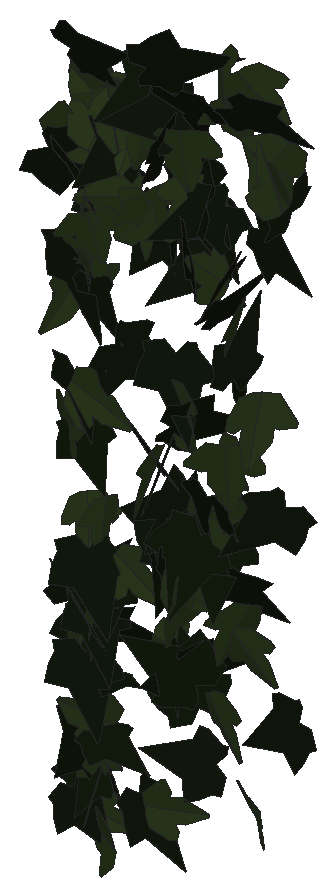
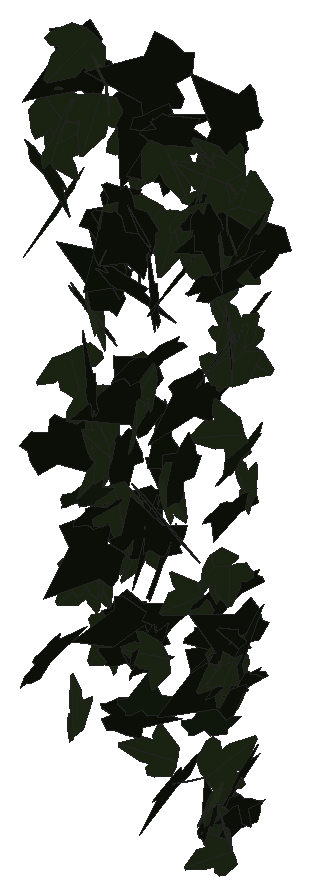
# SketchUp Ruby script. Lengths in inches.
U = 1.inch
M = Sketchup.active_model
def pt(a) = Geom::Point3d.new(a.map { |v| v * U })
def face(e, loops, mat)
  f = e.add_face(loops[0].map { |a| pt(a) })
  loops[1..].each { |l| e.add_face(l.map { |a| pt(a) }).erase! }
  f.material = f.back_material = mat if mat
  f
end
# faces: each face lists its corners as indices into pts; further lists are holes
def faces(e, pts, list, mat = nil) = list.each { |f| face(e, (f[0].is_a?(Array) ? f : [f]).map { |l| l.map { |i| pts[i] } }, mat) }
# xy, xz, yz: faces in a plane at the given z, y or x. An outline is a flat list of corners, or four numbers for a rectangle; further outlines are holes
def ring(l) = l.size == 4 ? [[l[0], l[1]], [l[2], l[1]], [l[2], l[3]], [l[0], l[3]]] : l.each_slice(2).to_a
def flat(e, list, mat, &to3) = list.each { |f| face(e, (f[0].is_a?(Array) ? f : [f]).map { |l| ring(l).map { |u, v| to3.(u, v) } }, mat) }
def xy(e, z, list, mat = nil) = flat(e, list, mat) { |x, y| [x, y, z] }
def xz(e, y, list, mat = nil) = flat(e, list, mat) { |x, z| [x, y, z] }
def yz(e, x, list, mat = nil) = flat(e, list, mat) { |y, z| [x, y, z] }
def lines(e, pts, list) = list.each { |a, b| e.add_line(pt(pts[a]), pt(pts[b])) }
# prism: a flat outline (further loops are holes) pulled along v
def prism(e, loops, v, mat = nil)
  f = face(e, loops, mat); d = Geom::Vector3d.new(v.map { |x| x * U })
  f.pushpull(f.normal.samedirection?(d) ? d.length : -d.length)
end
def box(e, o, s, mat = nil) = prism(e, [[o, [o[0] + s[0], o[1], o[2]], [o[0] + s[0], o[1] + s[1], o[2]], [o[0], o[1] + s[1], o[2]]]], [0, 0, s[2]], mat)
def at(x, y, z, deg = 0) = Geom::Transformation.translation(pt([x, y, z])) * Geom::Transformation.rotation(ORIGIN, Z_AXIS, deg.degrees)
def axes(o, x, y, z) = Geom::Transformation.new([*x, 0, *y, 0, *z, 0, *pt(o).to_a, 1])
def part(name) = M.definitions.add(name)
# library, detail: a bought-in or finely detailed component or shape, given as its bounding box
def library(name, o, s) = part(name).tap { |d| box(d.entities, o, s) }
def detail(e, o, s) = box(e.add_group.entities, o, s)
def put(e, d, t, mat = nil) = e.add_instance(d, t).tap { |i| i.material = mat if mat }
def group(e, t, mat = nil) = e.add_group.tap { |g| g.transformation = t; g.material = mat if mat }.entities
root = M.entities
M.materials.add("efeu1").color = [18, 25, 13]
M.materials.add("efeu2").color = [43, 57, 29]
c1 = part("ivyleaf_10")
p = [[0,0.5,-0.03],[-0.0625,2.02,-0.43],[-0.19,2.01,-0.46],[-0.54,1.05,-0.29],[-0.52,0.625,-0.18],[-0.83,0.76,-0.28],
  [-1.16,0.64,-0.33],[-1.15,0.33,-0.24],[-0.77,-0.39,0.02],[-0.3,-0.51,0.16],[0.04,-0.48,0.23],[-0.02,2.01,-0.4375],
  [-0.06,2.01,-0.43],[0.04,-0.49,0.23],[0.67,-0.49,0.14],[1.38,0.36,-0.2],[1.375,0.51,-0.24],[0.81,0.65,-0.19],
  [0.62,0.59,-0.15],[0.6,1.09,-0.28],[0.5,1.23,-0.31]]
faces(c1.entities,p,[[0,1,2,3,4,5,6,7,8,9,10],[11,12,0,13,14,15,16,17,18,19,20]],"efeu2")
c2 = part("ivyleaf_9")
p = [[1.54,2.16,1.25],[1.36,2.04,1.19],[-0.21,0.99,0.68],[-0.71,1.11,0.82],[-0.85,0.86,0.67],[-0.8,0.17,0.21],
  [-0.9,-0.01,0.1],[-0.67,-0.16,-0.02],[-0.08,-0.08,-0.05],[-0.03,-0.6,-0.4],[0.65,-0.88,-0.66],[0.83,-0.6,-0.49],
  [1.29,-0.42,-0.43],[1.8125,-0.07,-0.26],[1.21,0.44,0.15]]
faces(c2.entities,p,[[0,1,2,3,4,5,6,7,8,9,10,11,12,13,14]],"efeu1")
put(root,c1,axes([585.43,126.89,216.26],[0.20905,0.88225,-0.1568],[-0.02786,-0.15453,-0.90664],[-0.89564,0.21074,-0.00839]))
put(root,c1,axes([585.7,127.05,216.36],[-0.86933,0.26454,0.1104],[-0.10638,0.02961,-0.90868],[-0.26618,-0.87581,0.00262]))
put(root,c2,axes([586.2,127.75,234.65],[-0.4505,-1.00807,-0.18395],[-0.0756,-0.1677,1.10415],[-1.02192,0.4568,-0.00059]))
put(root,c1,axes([585.82,126.15,231.04],[0.26542,0.80579,-0.93729],[-0.44182,-0.83347,-0.84165],[-1.15439,0.50427,0.10662]))
put(root,c1,axes([586.16,127.11,211.16],[-0.42988,-0.39281,-0.89243],[-0.69049,-0.56599,0.58173],[-0.68844,0.81295,-0.02621]))
put(root,c2,axes([585.43,126.77,210.41],[-0.05024,-0.67641,0.89624],[-0.10277,-0.89061,-0.67792],[1.11814,-0.11225,-0.02203]))
put(root,c2,axes([585.53,126.99,215.375],[-0.24572,-0.87489,-0.04621],[0.01577,0.04356,-0.90873],[0.87597,-0.2462,0.0034]))
put(root,c2,axes([585.18,126.625,226.41],[0.33854,-0.96981,0.40729],[0.20018,-0.36064,-1.02513],[1.03264,0.38786,0.0652]))
put(root,c1,axes([585.7,126.66,230.41],[-0.41477,-1.0757,-0.15207],[-0.02291,-0.15408,1.1524],[-1.08615,0.41403,0.03377]))
put(root,c1,axes([585.64,126.8125,220.75],[0.5479,0.75565,-0.02304],[-0.01674,-0.01633,-0.93337],[-0.75581,0.54814,0.00396]))
put(root,c1,axes([585.18,126.07,224.39],[-0.45576,0.14929,0.94388],[0.90384,-0.27221,0.47948],[0.31029,1.01219,-0.01027]))
put(root,c2,axes([586.03,126.6875,215.52],[0.58846,-0.99171,0.4904],[-0.25923,0.41639,1.15312],[-1.07554,-0.64296,-0.00962]))
put(root,c2,axes([585.51,126.76,224.1],[0.1079,-0.87299,-0.38514],[-0.01408,0.3861,-0.8791],[0.95407,0.10443,0.03058]))
put(root,c2,axes([585.39,127.19,232.5],[-0.23152,-0.02001,-1.13527],[1.10371,-0.27602,-0.22022],[-0.2666,-1.12528,0.07421]))
put(root,c2,axes([585.27,125.92,236.77],[0.54697,-0.82406,0.44768],[0.24394,-0.3754,-0.98906],[0.90553,0.59889,-0.00397]))
put(root,c2,axes([585.26,125.15,237.09],[0.09927,0.31832,-1.30453],[0.49473,1.20741,0.33226],[1.24835,-0.50381,-0.02794]))
put(root,c2,axes([585.64,125.9,217.02],[-0.10869,-0.07593,1.08353],[0.91589,0.57898,0.13245],[-0.5839,0.92229,0.00606]))
put(root,c2,axes([586.07,126.57,209.21],[-0.52865,-0.66925,0.02633],[-0.01514,-0.02159,-0.85285],[0.6696,-0.52886,0.0015]))
put(root,c1,axes([585.75,126.25,231.91],[-0.81,-0.25854,0.56525],[0.53534,0.18165,0.85022],[-0.31586,0.97088,-0.00855]))
put(root,c1,axes([585.71,126.32,231.35],[-0.61315,0.22458,0.77909],[0.70857,-0.32642,0.65173],[0.39416,0.93615,0.04035]))
put(root,c1,axes([586.16,126.68,208.8],[0.65539,-0.82227,0.0305],[0.01965,-0.02334,-1.05151],[0.8226,0.65568,0.00082]))
put(root,c1,axes([585.98,126.27,216.35],[-0.35302,-0.53148,-0.79615],[0.41333,0.68076,-0.63772],[0.86342,-0.54319,-0.02023]))
put(root,c2,axes([585.52,125.85,232.41],[0.61194,-1.20843,0.05809],[0.0345,-0.04764,-1.35451],[1.20934,0.61284,0.00924]))
put(root,c1,axes([585.47,125.34,237.7],[-0.1941,-0.30638,1.14812],[0.86858,0.75731,0.34894],[-0.81093,0.88449,0.09894]))
put(root,c2,axes([586.75,127.12,237.64],[0.37189,0.07914,-1.04316],[-1.03126,-0.15844,-0.37967],[-0.17592,1.09607,0.02043]))
put(root,c2,axes([585.9,125.73,208.58],[0.27516,-0.71599,-0.67061],[-0.14859,0.65804,-0.76353],[0.96968,0.304,0.0733]))
put(root,c1,axes([586.15,127.01,209.59],[-0.04471,-0.90231,0.11582],[0.22003,-0.12324,-0.8752],[0.8827,-0.01499,0.22403]))
put(root,c1,axes([586.45,126.43,236.62],[0.21412,-1.02771,-0.08026],[-0.01363,0.07915,-1.04978],[1.03075,0.21454,0.00279]))
put(root,c1,axes([586.16,126.98,210.19],[0.54963,-0.61414,-0.27508],[0.28349,0.53344,-0.6245],[0.6103,0.3053,0.53783]))
put(root,c1,axes([585.85,126.98,207.12],[0.31525,0.16728,0.79766],[0.58161,0.55295,-0.34583],[-0.57093,0.65566,0.08814]))
put(root,c2,axes([585.91,126.64,215.5],[0.83714,0.54152,0.56986],[0.47909,0.30855,-0.99702],[-0.62325,0.96454,-0.00099]))
put(root,c1,axes([586.46,126.82,220.84],[-0.04804,-0.94628,0.20964],[0.23662,-0.215,-0.91624],[0.9399,0.00576,0.24138]))
put(root,c2,axes([586.42,126.95,217.52],[-0.52671,-0.6679,-0.42065],[0.24692,0.3409,-0.85045],[0.74971,-0.58151,-0.01542]))
put(root,c1,axes([586.29,126.48,216.25],[0.25401,-0.57922,0.64008],[0.49141,-0.45154,-0.60362],[0.70973,0.51994,0.18885]))
put(root,c2,axes([586.17,127.56,208.73],[0.07582,-0.31567,0.90545],[0.24981,-0.87041,-0.32437],[0.92578,0.26072,0.01337]))
put(root,c1,axes([586.32,125.86,236.46],[0.61511,-0.57118,0.55522],[0.45127,-0.32819,-0.83756],[0.6564,0.76087,0.05553]))
put(root,c2,axes([586.26,125.92,214.59],[0.02385,-1.17752,-0.17482],[0.11409,0.17631,-1.172],[1.18495,0.00672,0.11636]))
put(root,c1,axes([585.95,126.39,239.38],[-0.61446,-0.05872,1.09244],[1.08959,0.07974,0.61714],[-0.09831,1.25085,0.01194]))
put(root,c2,axes([586.35,126.11,231.22],[0.55401,-0.7372,-0.33447],[-0.18768,0.27729,-0.92203],[0.78747,0.58473,0.01555]))
put(root,c2,axes([586.41,127.43,213.2],[-0.40599,-0.70521,0.28275],[0.55914,-0.49437,-0.43018],[0.51442,-0.01921,0.69072]))
put(root,c2,axes([586.31,126.49,216.58],[0.10588,-1.10446,-0.09752],[0.10896,0.10785,-1.1032],[1.10339,0.09533,0.1183]))
put(root,c1,axes([585.87,126.5,239.27],[0.31865,0.07133,-1.18141],[1.16699,0.18511,0.32594],[0.19739,-1.20955,-0.01979]))
put(root,c2,axes([586.27,126.85,210.74],[0.41342,-0.70404,-0.30321],[0.36862,0.48464,-0.62272],[0.67211,0.16727,0.52803]))
put(root,c2,axes([585.93,125.57,241.57],[1.00706,0.17208,-0.72482],[0.68965,0.24555,1.01648],[0.28171,-1.21624,0.10267]))
put(root,c2,axes([586.5,125.85,219.3],[0.02332,-1.16152,-0.33366],[0.11175,0.33437,-1.15616],[1.20331,-0.00854,0.11384]))
put(root,c1,axes([587.66,125.53,206.9],[0.05311,-0.03825,-1.11885],[-0.76709,0.81459,-0.06426],[0.81539,0.76883,0.01242]))
put(root,c1,axes([587.06,125.21,234.53],[-0.82013,-0.69456,-0.20292],[0.15186,0.13467,-1.07471],[0.70748,-0.83406,-0.00455]))
put(root,c1,axes([587.08,126.42,239.85],[-0.55839,1.03577,-0.30731],[0.10192,-0.29389,-1.17571],[-1.07558,-0.56558,0.04813]))
put(root,c1,axes([586.92,125.65,238.03],[0.94405,0.559,-0.5015],[0.41893,0.27658,1.09691],[0.62328,-1.03259,0.02232]))
put(root,c1,axes([586.4375,125.47,226.58],[0.40141,0.08272,1.12506],[1.0697,0.35134,-0.40748],[-0.35827,1.14169,0.04388]))
put(root,c2,axes([587.63,126.76,237.56],[-0.4052,-0.74195,0.67552],[-0.34822,-0.57926,-0.8451],[0.94104,-0.53383,-0.02185]))
put(root,c1,axes([587.73,126.5,235.22],[0.02967,0.41781,1.12444],[-0.08277,-1.12139,0.41886],[1.1967,-0.08792,0.00109]))
put(root,c1,axes([587.5,127.3125,237.72],[-0.59019,-0.54327,0.56866],[0.41988,-0.81883,-0.3465],[0.66499,0.03485,0.72347]))
put(root,c2,axes([587.6875,126.12,228.76],[0.16175,-0.27011,-1.09009],[-0.25001,1.06504,-0.301],[1.09488,0.2831,0.09231]))
put(root,c1,axes([587.5625,126.66,218.77],[0.54458,0.21815,0.87221],[0.81158,0.31953,-0.58665],[-0.38689,0.97735,-0.00289]))
put(root,c2,axes([588.41,127.78,233.65],[-0.16887,-0.82216,0.83289],[-0.03253,-0.83789,-0.83369],[1.16987,-0.14197,0.09705]))
put(root,c1,axes([589.26,125.74,235.33],[0.82709,-0.43387,-0.77565],[-0.66843,0.39464,-0.9335],[0.58573,1.06301,0.02997]))
put(root,c2,axes([589.42,126.79,240.91],[-0.89036,-0.4522,0.43981],[-0.40068,-0.1822,-0.99846],[0.48722,-0.9762,-0.01738]))
put(root,c2,axes([588.1,126.95,224.42],[0.53651,-0.66735,0.79324],[0.5216,-0.59808,-0.85595],[0.89583,0.74791,0.02331]))
put(root,c1,axes([588.92,126.91,223.83],[0.41571,-0.94659,0.56429],[0.2117,-0.52327,-1.03375],[1.0815,0.46628,-0.01455]))
put(root,c2,axes([588.78,127.91,232.625],[-0.08967,0.25336,1.0693],[0.23268,-1.04415,0.26691],[1.07399,0.24737,0.03145]))
put(root,c1,axes([589.61,126.17,239.66],[-0.55352,-1.04932,0.43132],[-0.16101,-0.4024,-1.18559],[1.12302,-0.57488,0.04261]))
put(root,c1,axes([589.38,125.85,235.91],[-0.61043,-0.8753,-0.35463],[0.18505,0.30322,-1.06694],[0.9261,-0.63753,-0.02056]))
put(root,c2,axes([590.27,126.26,222.02],[-0.73579,0.70353,0.66675],[-0.51996,0.41997,-1.01694],[-0.81801,-0.89976,0.04668]))
put(root,c2,axes([589.09,125.82,209.37],[0.61425,-0.83268,-0.65475],[-0.31366,0.57996,-1.03181],[1.01177,0.68532,0.07764]))
put(root,c2,axes([589.42,127.97,213.36],[-0.37807,-0.72146,0.23514],[0.59936,-0.44504,-0.40179],[0.46536,-0.01294,0.70852]))
put(root,c1,axes([589.09,127.35,215.67],[-0.24574,-0.01065,-1.02888],[0.98071,-0.32245,-0.2309],[-0.31129,-1.00747,0.08478]))
put(root,c2,axes([590.78,126.04,240.08],[-0.60156,-0.20562,0.89498],[-0.74351,-0.51887,-0.61896],[0.53894,-0.94532,0.14506]))
put(root,c2,axes([589.56,126.49,219.57],[0.489,-0.30264,-1.07371],[0.94608,-0.50868,0.57425],[-0.59109,-1.06453,0.03085]))
put(root,c2,axes([590.21,126.58,220.27],[-0.83141,-0.2378,0.72787],[0.72279,0.11101,0.86188],[-0.25281,1.09941,0.07041]))
put(root,c2,axes([590.5,124.83,238.53],[0.13637,0.48472,1.09069],[0.34913,1.03357,-0.50299],[-1.14134,0.37408,-0.02354]))
put(root,c2,axes([590.875,124.28,224.36],[-0.00651,0.55823,1.15868],[0.03599,1.15832,-0.55786],[-1.28564,0.0296,-0.02148]))
put(root,c2,axes([590.59,126.79,214.72],[-0.19481,-0.26657,1.01239],[-0.39467,-0.93509,-0.32216],[0.96966,-0.43416,0.07227]))
put(root,c2,axes([590.78,125.33,221.3125],[0.41891,-0.2919,-1.07463],[-0.88307,0.61238,-0.51058],[0.67839,0.9774,-0.00104]))
put(root,c1,axes([590.93,126.34,225.77],[-0.24379,0.88332,-0.61648],[-0.14013,0.60069,0.91612],[1.06802,0.28044,-0.02052]))
put(root,c2,axes([591.32,127.54,233.46],[-1.17803,0.01297,0.11527],[-0.11592,-0.08817,-1.17473],[-0.00428,-1.18036,0.08902]))
put(root,c2,axes([591.62,126.58,236.26],[-0.55964,0.1314,-0.98465],[-0.98974,0.02282,0.56558],[0.08488,1.13234,0.10286]))
put(root,c1,axes([591.07,126.92,236.48],[0.96289,0.50198,-0.52091],[-0.48964,-0.18614,-1.08447],[-0.53252,1.07882,0.05526]))
put(root,c2,axes([590,125.27,242.3],[0.5609,0.11298,1.11735],[1.09821,0.20601,-0.57212],[-0.23486,1.23314,-0.00679]))
put(root,c2,axes([590.52,126.2,229.21],[0.00513,-1.21542,-0.23705],[0.06869,0.23697,-1.21351],[1.23642,-0.00812,0.0684]))
put(root,c2,axes([590.97,125.7,241.05],[1.01301,0.59065,-0.46052],[-0.43918,-0.15903,-1.17003],[-0.60669,1.10136,0.07802]))
put(root,c2,axes([590.32,127.44,237.03],[-0.31667,-0.24893,-1.15327],[1.04657,0.49202,-0.39358],[0.54471,-1.09006,0.08572]))
put(root,c2,axes([591.83,125.63,215.48],[-0.12674,0.15204,1.14733],[-1.15503,0.0567,-0.1351],[-0.07352,-1.15292,0.14466]))
put(root,c1,axes([590.31,125.29,209.49],[-0.11881,-0.0745,1.02824],[0.89415,0.50776,0.1401],[-0.51316,0.90199,0.00606]))
put(root,c2,axes([591.53,126.29,214.14],[-0.96792,-0.41752,0.2475],[0.22662,0.09952,1.05413],[-0.42921,0.9941,-0.00158]))
put(root,c1,axes([590.98,125.67,228.02],[-0.86762,0.5641,-0.45871],[0.3514,-0.29988,-1.03343],[-0.63651,-0.93447,0.05474]))
put(root,c1,axes([591.39,125.51,239.42],[-1.10398,-0.57475,-0.03307],[0.03397,0.00636,-1.24459],[0.57469,-1.10446,0.01004]))
put(root,c2,axes([592.02,126.58,211.51],[-0.4507,-0.50246,-0.75358],[-0.50949,-0.55528,0.67495],[-0.74885,0.68021,-0.00567]))
put(root,c1,axes([591.87,126.79,222.1],[-1.02114,-0.04034,0.60947],[-0.60798,-0.04683,-1.02175],[0.05863,-1.18827,0.01958]))
put(root,c2,axes([590.82,127.45,235.6875],[-0.38545,-0.24415,-1.10407],[0.96672,0.53392,-0.45557],[0.58655,-1.04042,0.02531]))
put(root,c1,axes([591.5,124.9,220.22],[-0.06894,0.86156,0.82187],[-0.11052,0.81506,-0.8637],[-1.18556,-0.12608,0.03272]))
put(root,c2,axes([591.25,125.88,215.97],[0.08337,0.46391,-0.91226],[0.05378,0.91203,0.4687],[1.02203,-0.08583,0.04975]))
put(root,c2,axes([592.22,126.91,236.14],[-0.09585,-0.0803,-1.11108],[-0.35804,-1.05379,0.10705],[-1.05487,0.36497,0.06462]))
put(root,c2,axes([592.11,124.88,235.28],[0.43672,-0.08954,-1.05895],[-1.04776,0.15523,-0.44523],[0.17776,1.1349,-0.02265]))
put(root,c2,axes([591.21,125.3125,226.8],[0.71329,0.48201,0.85894],[0.72087,0.46718,-0.8608],[-0.67116,1.01405,-0.0117]))
put(root,c1,axes([591.86,124.56,219.5],[0.074,-0.65887,-1.06764],[0.09506,1.06937,-0.65335],[1.25097,-0.04228,0.11281]))
put(root,c2,axes([591.78,126.02,221.7],[-0.59089,-1.02463,0.00589],[-0.0027,-0.00524,-1.1828],[1.02464,-0.59089,0.00028]))
put(root,c2,axes([592.125,126.875,221.59],[-0.42612,-1.07799,-0.26982],[0.15323,0.22922,-1.15777],[1.10063,-0.44927,0.05672]))
put(root,c2,axes([592.67,125.41,224.05],[0.70731,0.21544,-0.83386],[-0.81112,-0.19609,-0.73869],[-0.28952,1.07571,0.03234]))
put(root,c1,axes([592.5625,126.18,233.34],[-0.28143,0.80193,0.62741],[0.0395,-0.64185,0.8381],[1.01744,0.24674,0.14101]))
put(root,c1,axes([592.17,127.14,242.24],[-0.32195,0.00342,-1.03168],[0.4896,-0.95079,-0.15594],[-0.90812,-0.51382,0.28169]))
put(root,c1,axes([591.93,127.54,224.7],[-0.10695,0.14783,-1.10289],[0.81484,-0.74414,-0.17876],[-0.7578,-0.82101,-0.03656]))
put(root,c2,axes([592.23,127.83,227.14],[-0.13602,0.29039,1.02051],[0.2456,-0.99231,0.3151],[1.03221,0.27437,0.0595]))
put(root,c2,axes([592.89,125.56,232.96],[0.12181,0.64793,0.94157],[0.12132,0.93423,-0.65857],[-1.13651,0.16917,0.03062]))
put(root,c1,axes([592.73,126.91,240.9],[-0.69011,-0.76058,-0.31741],[0.20486,0.2427,-1.02694],[0.79829,-0.71979,-0.01087]))
put(root,c1,axes([592.8,127.16,231.59],[0.55836,-1.05143,0.14462],[0.07381,-0.12455,-1.19047],[1.05876,0.56317,0.00672]))
put(root,c2,axes([592.6875,128.15,222.36],[-0.54844,-0.5782,0.40846],[0.31419,-0.66183,-0.51498],[0.63438,-0.17208,0.60819]))
put(root,c2,axes([592.45,126.75,219.65],[1.06537,0.43481,0.20912],[0.19849,0.06704,-1.15062],[-0.43976,1.08363,-0.01273]))
put(root,c1,axes([593.07,125.76,223.08],[-0.11458,0.38946,1.08071],[-0.30104,1.03794,-0.40596],[-1.1086,-0.3221,-0.00146]))
put(root,c2,axes([592.625,125.78,231.92],[0.184,1.09586,-0.16465],[0.02529,0.16271,1.1112],[1.10787,-0.18572,0.00198]))
put(root,c1,axes([593.33,126.75,218.5],[-0.22056,-1.0161,0.43504],[-0.09667,-0.42418,-1.03976],[1.10108,-0.24078,-0.00415]))
put(root,c1,axes([593.35,125.84,225.95],[-1.04392,-0.67789,0.02379],[0.0289,-0.08806,-1.24148],[0.67769,-1.04047,0.08958]))
put(root,c1,axes([592.9,125.82,214.76],[-0.86466,0.48843,-0.58878],[0.48687,-0.33403,-0.9921],[-0.59007,-0.99133,0.04419]))
put(root,c2,axes([593.74,125.78,229.77],[-0.89997,0.70578,0.14142],[0.09487,-0.10814,1.14341],[0.71353,0.90458,0.02635]))
put(root,c1,axes([593.65,126.43,217.61],[-0.87044,0.13392,-0.62445],[0.61782,-0.09087,-0.88067],[-0.1618,-1.0674,-0.00337]))
put(root,c1,axes([594.22,126.72,228],[0.56888,1.03387,-0.28],[-0.20271,-0.2074,-1.17763],[-1.05176,0.59918,0.07552]))
put(root,c1,axes([595.26,126.49,238.01],[-0.68769,0.32757,-0.98954],[-0.89027,0.432,0.76171],[0.54213,1.12494,-0.00437]))
put(root,c1,axes([594.33,125.89,242.9375],[-0.91408,-0.28545,-0.69087],[0.66996,0.17123,-0.95716],[0.33157,-1.13293,0.02941]))
put(root,c1,axes([594.38,126.26,210.1],[-0.71837,0.20874,0.84062],[0.7268,-0.4488,0.73255],[0.47115,1.01059,0.15169]))
put(root,c2,axes([594.53,126.49,236],[0.84907,-0.57421,-0.6663],[-0.4319,0.53459,-1.01108],[0.76625,0.9376,0.16842]))
put(root,c2,axes([595.41,126.68,223.95],[0.07661,0.15798,-1.08843],[-0.34183,-1.03361,-0.17408],[-1.04537,0.34957,-0.02284]))
put(root,c1,axes([595.4,126.67,239.86],[-0.7057,-0.58402,0.64235],[-0.41727,-0.49775,-0.91096],[0.7613,-0.81418,0.09615]))
put(root,c2,axes([595.64,126.85,237.17],[-0.45742,0.81924,0.50508],[-0.32637,0.39405,-0.93472],[-0.9054,-0.55594,0.08177]))
put(root,c2,axes([594.96,128.12,213.66],[0.29166,-0.70234,-0.78555],[0.31645,-0.71908,0.7604],[-1.0051,-0.43021,0.01145]))
put(root,c2,axes([594.38,125.17,241.99],[1.11225,0.3174,0.36285],[0.35131,0.09115,-1.15662],[-0.33012,1.16638,-0.00835]))
put(root,c1,axes([595.17,126.54,237.76],[-0.15443,1.23428,0.10625],[0.0129,-0.10547,1.2439],[1.23878,0.15497,0.00029]))
